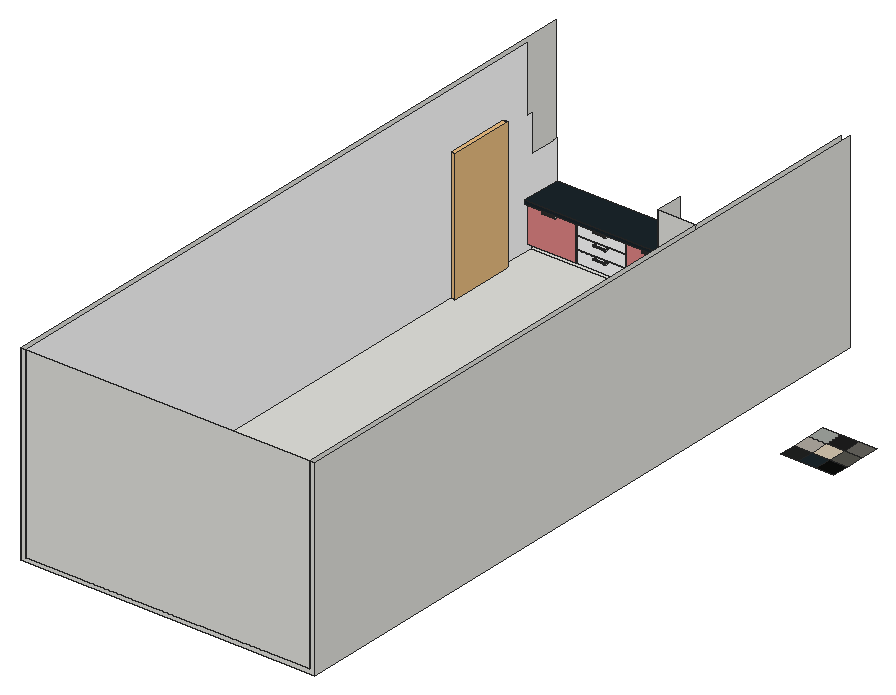
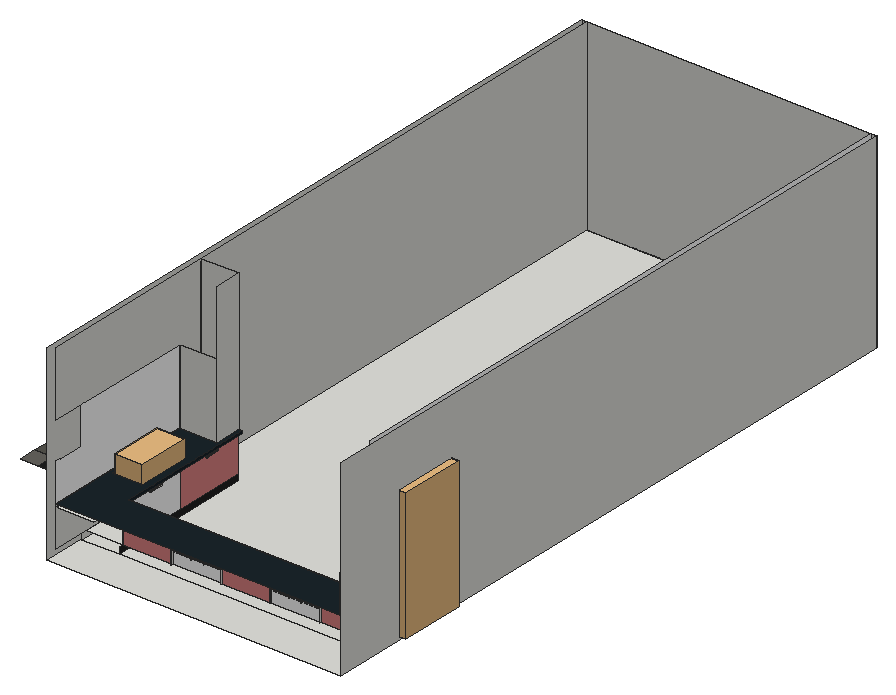
# SketchUp Ruby script. Lengths in inches.
U = 1.inch
M = Sketchup.active_model
def pt(a) = Geom::Point3d.new(a.map { |v| v * U })
def face(e, loops, mat)
  f = e.add_face(loops[0].map { |a| pt(a) })
  loops[1..].each { |l| e.add_face(l.map { |a| pt(a) }).erase! }
  f.material = f.back_material = mat if mat
  f
end
# faces: each face lists its corners as indices into pts; further lists are holes
def faces(e, pts, list, mat = nil) = list.each { |f| face(e, (f[0].is_a?(Array) ? f : [f]).map { |l| l.map { |i| pts[i] } }, mat) }
# xy, xz, yz: faces in a plane at the given z, y or x. An outline is a flat list of corners, or four numbers for a rectangle; further outlines are holes
def ring(l) = l.size == 4 ? [[l[0], l[1]], [l[2], l[1]], [l[2], l[3]], [l[0], l[3]]] : l.each_slice(2).to_a
def flat(e, list, mat, &to3) = list.each { |f| face(e, (f[0].is_a?(Array) ? f : [f]).map { |l| ring(l).map { |u, v| to3.(u, v) } }, mat) }
def xy(e, z, list, mat = nil) = flat(e, list, mat) { |x, y| [x, y, z] }
def xz(e, y, list, mat = nil) = flat(e, list, mat) { |x, z| [x, y, z] }
def yz(e, x, list, mat = nil) = flat(e, list, mat) { |y, z| [x, y, z] }
def lines(e, pts, list) = list.each { |a, b| e.add_line(pt(pts[a]), pt(pts[b])) }
# prism: a flat outline (further loops are holes) pulled along v
def prism(e, loops, v, mat = nil)
  f = face(e, loops, mat); d = Geom::Vector3d.new(v.map { |x| x * U })
  f.pushpull(f.normal.samedirection?(d) ? d.length : -d.length)
end
def box(e, o, s, mat = nil) = prism(e, [[o, [o[0] + s[0], o[1], o[2]], [o[0] + s[0], o[1] + s[1], o[2]], [o[0], o[1] + s[1], o[2]]]], [0, 0, s[2]], mat)
def at(x, y, z, deg = 0) = Geom::Transformation.translation(pt([x, y, z])) * Geom::Transformation.rotation(ORIGIN, Z_AXIS, deg.degrees)
def axes(o, x, y, z) = Geom::Transformation.new([*x, 0, *y, 0, *z, 0, *pt(o).to_a, 1])
def part(name) = M.definitions.add(name)
# library, detail: a bought-in or finely detailed component or shape, given as its bounding box
def library(name, o, s) = part(name).tap { |d| box(d.entities, o, s) }
def detail(e, o, s) = box(e.add_group.entities, o, s)
def put(e, d, t, mat = nil) = e.add_instance(d, t).tap { |i| i.material = mat if mat }
def group(e, t, mat = nil) = e.add_group.tap { |g| g.transformation = t; g.material = mat if mat }.entities
root = M.entities
M.materials.add("Generic").color = [255, 255, 255]
M.materials.add("Generic\#1").color = [224, 133, 133]
M.materials.add("Marble (16)").color = [160, 165, 159]
M.materials.add("Marble (17)").color = [30, 30, 30]
M.materials.add("Marble (18)").color = [102, 99, 94]
M.materials.add("Marble (19)").color = [84, 83, 77]
M.materials.add("Marble (23)").color = [175, 169, 160]
M.materials.add("Marble (24)").color = [211, 197, 174]
M.materials.add("Marble (25)").color = [13, 14, 12]
M.materials.add("Marble (27)").color = [27, 37, 43]
M.materials.add("Marble (28)").color = [33, 34, 33]
M.materials.add("[0136_Charcoal]").color = [35, 35, 35]
M.materials.add("[Color M00]").color = [255, 255, 255]
c1 = part("Group\#105")
prism(c1.entities,[[[0.55,0,1.11],[0.51,0,1.03],[0.44,0,0.97],[0.36,0,0.9375],[0.28,0,0.92],[0.19,0,0.9375],[0.11,0,0.97],[0.05,0,1.03],[0,0,1.11],[0,0,0],[0.55,0,0]]],[0,0.79,0])
c2 = part("Cabinet bar pull")
put(c2.entities,c1,axes([0,1.42,1.36],[0,0,-1],[1,0,0],[0,-1,0]))
g1 = group(c2.entities,at(0,1.42,1.36))
prism(g1,[[[0,-1.28,-0.57],[0,-1.32,-0.53],[0,-1.35,-0.49],[0,-1.38,-0.4375],[0,-1.4,-0.39],[0,-1.41,-0.33],[0,-1.42,-0.28],[0,-1.41,-0.22],[0,-1.4,-0.17],[0,-1.38,-0.11],[0,-1.35,-0.0625],[0,-1.32,-0.02],[0,-1.28,0.02],[0,-1.19,0.02],[0,-1.11,0],[0,-1.03,-0.05],[0,-0.97,-0.11],[0,-0.9375,-0.19],[0,-0.92,-0.28],[0,-0.9375,-0.36],[0,-0.97,-0.44],[0,-1.03,-0.51],[0,-1.11,-0.55],[0,-1.19,-0.57]]],[13.07,0,0])
put(c2.entities,c1,axes([12.28,1.42,1.36],[0,0,-1],[1,0,0],[0,-1,0]))
c3 = part("23")
xy(c3.entities,0,[[0,22.83,11.42,34.25]],"Marble (16)")
xy(c3.entities,0,[[11.42,22.83,22.83,34.25]],"Marble (17)")
xy(c3.entities,0,[[22.83,22.83,34.25,34.25]],"Marble (18)")
xy(c3.entities,0,[[22.83,11.42,34.25,22.83]],"Marble (19)")
xy(c3.entities,0,[[0,11.42,11.42,22.83]],"Marble (23)")
xy(c3.entities,0,[[11.42,11.42,22.83,22.83]],"Marble (24)")
xy(c3.entities,0,[[22.83,0,34.25,11.42]],"Marble (25)")
xy(c3.entities,0,[[11.42,0,22.83,11.42]],"Marble (27)")
xy(c3.entities,0,[[0,0,11.42,11.42]],"Marble (28)")
c4 = library("door (1)",[38.93,25.48,0],[40,9.94,82.68])
c5 = library("Component_12",[0,0,0],[17.72,31.5,20.63])
xy(root,0,[[4.74,0,194.24,431]])
xy(root,2.5625,[[7.99,0,191,0,191,311,167,311,167,406.75,7.99,406.75,7.99,384.54,4.74,384.54,4.74,342.29,7.99,342.29],[167,311,191,406.75]])
xy(root,6.5625,[[167,311,167.56,357.08],[167.56,311,190.94,357.08],[190.94,311,191,357.08],[167,357.08,167.56,357.38],[167.56,357.08,190.94,357.38],
  [190.94,357.08,191,357.38],[167,357.38,190.94,403.75],[190.94,357.38,191,403.75]])
xy(root,14.5625,[[40.09,403.75,71.59,404.32],[103.69,403.75,135.2,404.32]])
xy(root,14.86,[[40.09,403.75,71.59,404.32],[103.69,403.75,135.2,404.32]])
xy(root,22.5625,[[40.09,403.75,71.59,404.32],[103.69,403.75,135.2,404.32]])
xy(root,22.86,[[40.09,403.75,71.59,404.32],[103.69,403.75,135.2,404.32]])
xy(root,30.5625,[[165,311,165,403.75,167,403.75,167,357.38,167.56,357.38,167.56,357.08,167,357.08,167,311],[[167,311,167,357.08,167.56,357.08,167.56,357.38,167,357.38,167,427.75,190.94,427.75,190.94,311],[169.58,351.49,188.46,384.99]],[190.94,311,191,427.75],[7.99,401.75,7.99,403.75,39.79,403.75,39.79,404.32,40.09,404.32,40.09,403.75,71.59,403.75,71.59,404.32,71.89,404.32,71.89,403.75,103.39,403.75,103.39,404.32,103.69,404.32,103.69,403.75,135.2,403.75,135.2,404.32,135.5,404.32,135.5,403.75,165,403.75,165,401.75]])
xy(root,32.5625,[[[165,311,166.97,311,166.97,328.41,191,328.41,191,427.75,7.99,427.75,7.99,401.75,165,401.75],[169.58,351.49,188.46,384.99]]],"Marble (27)")
xz(root,0,[[4.74,0,194.24,0,194.24,122.5625,191,122.5625,191,2.5625,7.99,2.5625,7.99,122.5625,4.74,122.5625],[7.99,2.5625,191,122.5625]])
xz(root,311,[[167,2.5625,191,6.5625],[167,6.5625,190.94,30.5625],[190.94,6.5625,191,30.5625],[166.97,32.5625,191,122.5625]])
xz(root,311,[[165,30.5625,191,32.5625]],"Marble (27)")
xz(root,328.41,[[166.97,32.5625,191,80.5625]])
xz(root,342.29,[[4.74,2.5625,7.99,86.5625]])
xz(root,351.49,[[169.58,30.5625,188.46,32.5625]],"Marble (27)")
xz(root,357.08,[[167,6.5625,167.56,30.5625]])
xz(root,357.38,[[167,6.5625,167.56,30.5625]])
xz(root,384.54,[[4.74,2.5625,7.99,86.5625]])
xz(root,384.99,[[169.58,30.5625,188.46,32.5625]],"Marble (27)")
xz(root,401.75,[[7.99,30.5625,165,32.5625]],"Marble (27)")
xz(root,403.75,[[40.09,6.5625,71.59,14.5625],[103.69,6.5625,135.2,14.5625],[40.09,14.86,71.59,22.5625],[103.69,14.86,135.2,22.5625],[40.09,22.86,71.59,30.5625],
  [103.69,22.86,135.2,30.5625]],"Generic")
xz(root,403.75,[[7.99,6.5625,39.79,30.5625],[71.89,6.5625,103.39,30.5625],[135.5,6.5625,167,30.5625]],"Generic\#1")
yz(root,4.74,[[[0,0,431,122.5625],[342.29,2.5625,384.54,86.5625]]])
yz(root,7.99,[[0,2.5625,342.29,2.5625,342.29,86.5625,384.54,86.5625,384.54,2.5625,406.75,2.5625,406.75,6.5625,403.75,6.5625,403.75,30.5625,401.75,30.5625,401.75,32.5625,427.75,32.5625,427.75,56.97,425.57,56.97,425.57,56.6,407.75,56.6,407.75,80.5625,403.75,80.5625,403.75,122.5625,0,122.5625]],"[Color M00]")
yz(root,39.79,[[403.75,6.5625,404.32,30.5625]])
yz(root,40.09,[[403.75,6.5625,404.32,14.5625],[403.75,14.86,404.32,22.5625],[403.75,22.86,404.32,30.5625]])
yz(root,71.59,[[403.75,6.5625,404.32,14.5625],[403.75,14.86,404.32,22.5625]])
yz(root,71.89,[[403.75,6.5625,404.32,30.5625]])
yz(root,103.39,[[403.75,6.5625,404.32,30.5625]])
yz(root,103.69,[[403.75,6.5625,404.32,14.5625],[403.75,14.86,404.32,22.5625],[403.75,22.86,404.32,30.5625]])
yz(root,135.2,[[403.75,6.5625,404.32,14.5625],[403.75,14.86,404.32,22.5625]])
yz(root,135.5,[[403.75,6.5625,404.32,30.5625]])
yz(root,165,[[311,30.5625,401.75,32.5625]],"Marble (27)")
yz(root,166.97,[[311,32.5625,328.41,122.5625]])
yz(root,167,[[311,6.5625,357.08,30.5625]],"Generic\#1")
yz(root,167,[[311,2.5625,406.75,6.5625]],"[0136_Charcoal]")
yz(root,167,[[357.38,6.5625,403.75,30.5625]],"[Color M00]")
yz(root,167.56,[[357.08,6.5625,357.38,30.5625]])
yz(root,169.58,[[351.49,30.5625,384.99,32.5625]],"Marble (27)")
yz(root,188.46,[[351.49,30.5625,384.99,32.5625]],"Marble (27)")
yz(root,190.94,[[311,6.5625,427.75,30.5625]])
yz(root,191,[[0,2.5625,311,122.5625],[311,2.5625,406.75,6.5625],[311,6.5625,427.75,30.5625],[311,30.5625,427.75,32.5625],[311,32.5625,311,122.5625,427.75,122.5625,427.75,80.5625,328.41,80.5625,328.41,32.5625]])
yz(root,191,[[328.41,32.5625,328.41,80.5625,407.75,80.5625,407.75,56.6,425.07,56.6,425.07,57.16,427.75,57.16,427.75,32.5625]],"[Color M00]")
yz(root,194.24,[[0,0,431,122.5625]])
put(root,c2,axes([165.35,337.9375,27.68],[0,-0.6547,0],[1.16,0,0],[0,0,1.16]))
put(root,c3,at(235.41,323.97,0))
put(root,c4,axes([39.3125,301.17,2.23],[0,1.05625,0],[-1.11,0,0],[0,0,1.02]))
put(root,c5,axes([187.25,385.36,23.0625],[-1,0,0],[0,-1.0864,0],[0,0,1]))
put(root,c2,axes([165.35,383.25,27.68],[0,-0.6547,0],[1.16,0,0],[0,0,1.16]))
put(root,c2,axes([114.74,402.11,12.26],[0.6547,0,0],[0,1.16,0],[0,0,1.16]))
put(root,c2,axes([114.74,402.11,20.14],[0.6547,0,0],[0,1.16,0],[0,0,1.16]))
put(root,c2,axes([148.07,402.11,27.75],[0.6547,0,0],[0,1.16,0],[0,0,1.16]))
put(root,c2,axes([19.12,402.11,27.76],[0.6547,0,0],[0,1.16,0],[0,0,1.16]))
put(root,c2,axes([83.24,402.11,27.76],[0.6547,0,0],[0,1.16,0],[0,0,1.16]))
put(root,c2,axes([114.74,402.11,27.76],[0.6547,0,0],[0,1.16,0],[0,0,1.16]))
put(root,c2,axes([51.77,402.11,12.46],[0.6547,0,0],[0,1.16,0],[0,0,1.16]))
put(root,c2,axes([51.77,402.11,20.21],[0.6547,0,0],[0,1.16,0],[0,0,1.16]))
put(root,c2,axes([51.77,402.11,28.21],[0.6547,0,0],[0,1.16,0],[0,0,1.16]))
